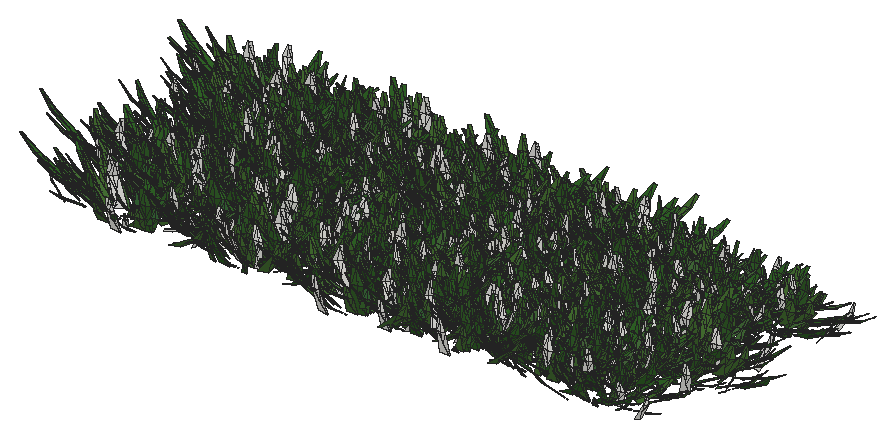
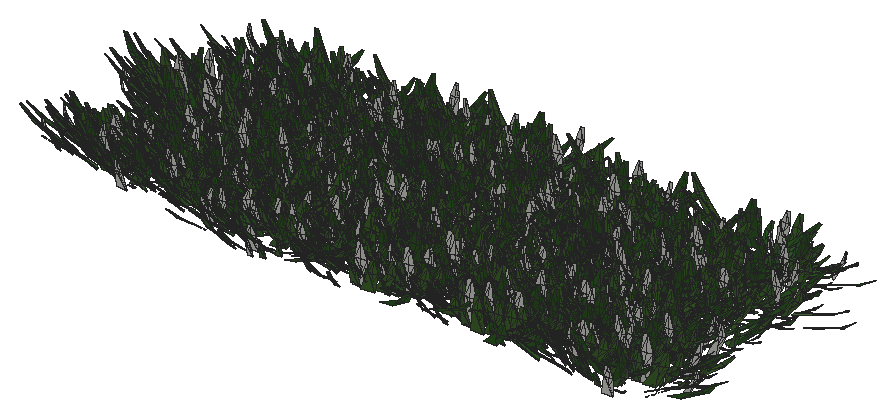
# SketchUp Ruby script. Lengths in inches.
U = 1.inch
M = Sketchup.active_model
def pt(a) = Geom::Point3d.new(a.map { |v| v * U })
def face(e, loops, mat)
  f = e.add_face(loops[0].map { |a| pt(a) })
  loops[1..].each { |l| e.add_face(l.map { |a| pt(a) }).erase! }
  f.material = f.back_material = mat if mat
  f
end
# faces: each face lists its corners as indices into pts; further lists are holes
def faces(e, pts, list, mat = nil) = list.each { |f| face(e, (f[0].is_a?(Array) ? f : [f]).map { |l| l.map { |i| pts[i] } }, mat) }
# xy, xz, yz: faces in a plane at the given z, y or x. An outline is a flat list of corners, or four numbers for a rectangle; further outlines are holes
def ring(l) = l.size == 4 ? [[l[0], l[1]], [l[2], l[1]], [l[2], l[3]], [l[0], l[3]]] : l.each_slice(2).to_a
def flat(e, list, mat, &to3) = list.each { |f| face(e, (f[0].is_a?(Array) ? f : [f]).map { |l| ring(l).map { |u, v| to3.(u, v) } }, mat) }
def xy(e, z, list, mat = nil) = flat(e, list, mat) { |x, y| [x, y, z] }
def xz(e, y, list, mat = nil) = flat(e, list, mat) { |x, z| [x, y, z] }
def yz(e, x, list, mat = nil) = flat(e, list, mat) { |y, z| [x, y, z] }
def lines(e, pts, list) = list.each { |a, b| e.add_line(pt(pts[a]), pt(pts[b])) }
# prism: a flat outline (further loops are holes) pulled along v
def prism(e, loops, v, mat = nil)
  f = face(e, loops, mat); d = Geom::Vector3d.new(v.map { |x| x * U })
  f.pushpull(f.normal.samedirection?(d) ? d.length : -d.length)
end
def box(e, o, s, mat = nil) = prism(e, [[o, [o[0] + s[0], o[1], o[2]], [o[0] + s[0], o[1] + s[1], o[2]], [o[0], o[1] + s[1], o[2]]]], [0, 0, s[2]], mat)
def at(x, y, z, deg = 0) = Geom::Transformation.translation(pt([x, y, z])) * Geom::Transformation.rotation(ORIGIN, Z_AXIS, deg.degrees)
def axes(o, x, y, z) = Geom::Transformation.new([*x, 0, *y, 0, *z, 0, *pt(o).to_a, 1])
def part(name) = M.definitions.add(name)
# library, detail: a bought-in or finely detailed component or shape, given as its bounding box
def library(name, o, s) = part(name).tap { |d| box(d.entities, o, s) }
def detail(e, o, s) = box(e.add_group.entities, o, s)
def put(e, d, t, mat = nil) = e.add_instance(d, t).tap { |i| i.material = mat if mat }
def group(e, t, mat = nil) = e.add_group.tap { |g| g.transformation = t; g.material = mat if mat }.entities
root = M.entities
M.materials.add("Material82").color = [68, 110, 58]
M.materials.add("Material83").color = [48, 90, 38]
M.materials.add("Material84").color = [68, 110, 48]
M.materials.add("Material85").color = [48, 90, 48]
M.materials.add("Material86").color = [58, 110, 58]
M.materials.add("Material87").color = [58, 90, 38]
M.materials.add("Material88").color = [68, 100, 58]
M.materials.add("Material89").color = [48, 100, 38]
c1 = part("grass00")
p = [[-0.6875,0.15,0],[-0.56,0.08,5.52],[-0.04,0.03,2.76],[0.48,-0.02,0],[0.35,-0.02,5.52],[-0.1,-0.14,5.52],
  [-0.12,0.65,8.37],[-0.42,0.65,8.37]]
faces(c1.entities,p,[[0,1,2,3],[3,2,4],[1,5,2],[5,4,2],[1,6,5],[4,5,6],[7,6,1]])
c2 = part("Group16\#1")
put(c2.entities,c1,axes([1.44,-0.61,-0.01],[0.05352,0.12609,0],[-0.10704,0.04543,0.07239],[0.06664,-0.02828,0.11628]),"Material85")
put(c2.entities,c1,axes([0.76,-0.15,-0.01],[0.04676,0.24062,0],[-0.23162,0.04501,0.06642],[0.0652,-0.01267,0.23595]),"Material82")
put(c2.entities,c1,axes([0.79,0.01,-0.01],[-0.00606,0.34651,0],[-0.34381,-0.00602,0.0432],[0.04319,0.00076,0.34386]))
put(c2.entities,c1,axes([1,0.23,-0.01],[-0.07192,0.31144,0],[-0.28722,-0.06632,0.1236],[0.12043,0.02781,0.29478]),"Material84")
put(c2.entities,c1,axes([1.66,0.77,-0.01],[-0.13828,0.29651,0],[-0.21551,-0.1005,0.22471],[0.20365,0.09498,0.23779]),"Material89")
put(c2.entities,c1,axes([0.6875,0.52,-0.01],[-0.18126,0.24051,0],[-0.22746,-0.17142,0.09788],[0.07817,0.05891,0.28481]),"Material84")
put(c2.entities,c1,axes([0.68,0.78,-0.01],[-0.215,0.18688,0],[-0.12385,-0.14248,0.21334],[0.13995,0.16101,0.18878]),"Material82")
put(c2.entities,c1,axes([0.56,1,-0.01],[-0.13756,0.07624,0],[-0.06159,-0.11112,0.0927],[0.04494,0.08108,0.12705]),"Material84")
put(c2.entities,c1,axes([0.2,0.64,-0.01],[-0.23729,0.07254,0],[-0.05711,-0.18681,0.153],[0.04473,0.14632,0.19535]),"Material89")
put(c2.entities,c1,axes([0.0625,0.72,-0.01],[-0.28874,0.02525,0],[-0.02179,-0.24916,0.14647],[0.01276,0.14591,0.25012]),"Material82")
put(c2.entities,c1,axes([-0.08,0.62,-0.01],[-0.34089,-0.04187,0],[0.03255,-0.26504,0.216],[-0.02633,0.21439,0.26703]),"Material89")
put(c2.entities,c1,axes([-0.34,0.98,-0.01],[-0.14314,-0.0493,0],[0.04397,-0.12769,0.06843],[-0.02228,0.0647,0.13505]),"Material89")
put(c2.entities,c1,axes([-0.87,1.45,-0.01],[-0.23488,-0.14114,0],[0.13761,-0.22901,0.06087],[-0.03135,0.05217,0.26717]))
put(c2.entities,c1,axes([-0.72,0.77,-0.01],[-0.14208,-0.13251,0],[0.07209,-0.0773,0.16301],[-0.11118,0.11922,0.1057]),"Material89")
put(c2.entities,c1,axes([-0.62,0.43,-0.01],[-0.14845,-0.21203,0],[0.18654,-0.13061,0.12304],[-0.10079,0.07057,0.22772]),"Material82")
put(c2.entities,c1,axes([-0.68,0.29,-0.01],[-0.13639,-0.32136,0],[0.31723,-0.13464,0.05579],[-0.05136,0.0218,0.34462]),"Material83")
put(c2.entities,c1,axes([-0.64,0.125,-0.01],[-0.0458,-0.23569,0],[0.22124,-0.043,0.08276],[-0.08124,0.01579,0.22538]),"Material86")
put(c2.entities,c1,axes([-1.6,-0.03,-0.01],[0.00576,-0.32897,0],[0.27526,0.00482,0.18018],[-0.18015,-0.00315,0.2753]),"Material84")
put(c2.entities,c1,axes([-1.36,-0.31,-0.01],[0.05718,-0.24765,0],[0.18172,0.04196,0.17267],[-0.16825,-0.03885,0.1865]),"Material89")
put(c2.entities,c1,axes([-1.54,-0.72,-0.01],[0.06537,-0.14017,0],[0.13555,0.06321,0.03939],[-0.0357,-0.01665,0.14956]))
put(c2.entities,c1,axes([-1.19,-0.9,-0.01],[0.09597,-0.12735,0],[0.11214,0.08451,0.07557],[-0.06035,-0.04548,0.14042]),"Material88")
put(c2.entities,c1,axes([-0.47,-0.54,-0.01],[0.11588,-0.10072,0],[0.0618,0.0711,0.12124],[-0.07953,-0.0915,0.0942]))
put(c2.entities,c1,axes([-0.47,-0.84,-0.01],[0.11927,-0.0661,0],[0.06603,0.11913,0.00646],[-0.00313,-0.00565,0.13621]),"Material84")
put(c2.entities,c1,axes([-0.38,-1.24,-0.01],[0.28037,-0.08571,0],[0.0618,0.20215,0.20315],[-0.05939,-0.19428,0.21139]),"Material88")
put(c2.entities,c1,axes([-0.06,-0.66,-0.01],[0.22719,-0.01987,0],[0.01247,0.14255,0.17758],[-0.01547,-0.17691,0.1431]),"Material87")
put(c2.entities,c1,axes([0.11,-0.89,-0.01],[0.14882,0.01828,0],[-0.01058,0.08611,0.12229],[0.01491,-0.12138,0.08676]),"Material85")
put(c2.entities,c1,axes([0.25,-0.72,-0.01],[0.20481,0.07053,0],[-0.06206,0.18022,0.10291],[0.03351,-0.0973,0.1906]),"Material85")
put(c2.entities,c1,axes([0.85,-1.42,-0.01],[0.16481,0.09904,0],[-0.09472,0.15762,0.05616],[0.02893,-0.04814,0.18389]),"Material84")
put(c2.entities,c1,axes([1.01,-1.09,-0.01],[0.21858,0.20385,0],[-0.17495,0.1876,0.15339],[0.10462,-0.11218,0.25652]),"Material89")
put(c2.entities,c1,axes([1.01,-0.71,-0.01],[0.08733,0.12473,0],[-0.06445,0.04512,0.13037],[0.1068,-0.07477,0.07867]),"Material85")
c3 = part("Group15\#1")
put(c3.entities,c2,at(0,0,0))
c4 = part("3darcstudiotree_grass00\#1")
put(c4.entities,c3,at(0,0,0))
put(root,c4,axes([705.6875,346.47,-34.17],[-3.11874,1.35551,0],[-2.91461,-1.04296,-0.0082],[-0.03562,-0.01275,1.73071]))
put(root,c4,axes([707,353.64,-34.17],[-3.23633,-0.50825,0],[1.72306,-1.70642,-0.01803],[0.03469,-0.03435,1.81493]))
put(root,c4,axes([705.92,365.84,-34.17],[-1.77081,1.15286,0],[-3.98211,-0.9513,-0.05645],[-0.27396,-0.06545,1.97994]))
put(root,c4,axes([705.78,364.16,-34.17],[2.97915,0.86965,0],[-2.38175,1.26898,-0.05487],[-0.15774,0.08404,1.44987]))
put(root,c4,axes([707,361.99,-34.17],[3.36447,-1.00796,0],[2.1967,1.14039,-0.03309],[0.10605,0.05506,1.44206]))
put(root,c4,axes([708.45,350.61,-34.17],[-3.57677,-1.09741,0],[2.84767,-1.44352,-0.06227],[0.15089,-0.07649,1.37168]))
put(root,c4,axes([707.32,340.29,-34.17],[-0.9025,1.72738,0],[-3.54084,-0.28772,-0.03296],[-0.16809,-0.01366,1.411]))
put(root,c4,axes([707.48,359.44,-34.17],[-1.59741,1.49736,0],[-3.22806,-0.5356,-0.02216],[-0.12937,-0.02146,1.66252]))
put(root,c4,axes([708.26,348.21,-34.17],[-0.7508,1.54691,0],[-4.43091,-0.33447,-0.01652],[-0.07223,-0.00545,1.50529]))
put(root,c4,axes([708.45,368.2,-34.17],[4.00478,-0.12141,0],[0.32544,1.66956,-0.03486],[0.01415,0.07259,1.68524]))
put(root,c4,axes([708.85,357.11,-34.17],[3.83024,1.03121,0],[-2.22146,1.2833,-0.02215],[-0.08012,0.04629,1.8946]))
put(root,c4,axes([711.74,353.15,-34.17],[-3.68156,-0.36216,0],[0.87025,-1.37591,-0.04204],[0.06138,-0.09705,1.62585]))
put(root,c4,axes([711.4,339.76,-34.17],[-3.79448,1.12109,0],[-2.55555,-1.34526,-0.03017],[-0.0978,-0.05148,1.72726]))
put(root,c4,axes([711.77,363.96,-34.17],[-3.10715,1.0196,0],[-2.89034,-1.36991,-0.01948],[-0.06651,-0.03152,1.80807]))
put(root,c4,axes([711.98,361.45,-34.17],[3.31286,-0.55128,0],[1.80617,1.68812,-0.0407],[0.06877,0.06427,1.51351]))
put(root,c4,axes([711.25,342.87,-34.17],[3.22227,0.82324,0],[-2.17222,1.32236,-0.01048],[-0.0296,0.01802,1.55517]))
put(root,c4,axes([713.39,359.76,-34.17],[-4.269,-0.81813,0],[1.88917,-1.53314,-0.01545],[0.03796,-0.03081,1.8215]))
put(root,c4,axes([712.1,355.12,-34.17],[0.15057,1.31453,0],[-3.70176,0.06595,-0.0329],[-0.23461,0.00418,1.98251]))
put(root,c4,axes([712.07,347.21,-34.17],[-0.68682,1.71759,0],[-4.33467,-0.26958,-0.03641],[-0.15889,-0.00988,1.45326]))
put(root,c4,axes([712.49,348.04,-34.17],[-1.33529,1.77622,0],[-3.16975,-0.37061,-0.00114],[-0.00828,-0.00097,1.86907]))
put(root,c4,axes([712.03,356.7,-34.17],[1.34239,1.63135,0],[-4.02681,0.51535,-0.01715],[-0.07258,0.00929,1.41194]))
put(root,c4,axes([713.12,366.09,-34.17],[-1.89402,1.2029,0],[-3.60721,-0.88336,-0.02009],[-0.09037,-0.02213,1.68525]))
put(root,c4,axes([714.06,350.73,-34.17],[2.81192,0.87479,0],[-2.84329,1.42145,-0.06164],[-0.14998,0.07498,1.3518]))
put(root,c4,axes([714.39,344.07,-34.17],[0.48103,1.53156,0],[-4.51259,0.22043,-0.03401],[-0.13914,0.0068,1.40523]))
put(root,c4,axes([716.875,360.96,-34.17],[-3.65599,0.07986,0],[-0.21877,-1.55768,-0.04105],[-0.01403,-0.0999,1.83253]))
put(root,c4,axes([717.49,350.74,-34.17],[-2.36391,-1.30666,0],[2.88424,-0.81154,-0.04134],[0.24623,-0.06928,1.943]))
put(root,c4,axes([716.77,345.07,-34.17],[-2.91503,0.96344,0],[-2.99535,-1.40954,-0.01682],[-0.05566,-0.02619,1.80026]))
put(root,c4,axes([717.57,349.41,-34.17],[2.5477,-1.31265,0],[2.99582,0.90433,-0.00025],[0.00104,0.00031,1.45509]))
put(root,c4,axes([717.4,363.8125,-34.17],[2.84002,-1.42543,0],[3.17904,0.98511,-0.04001],[0.1906,0.05906,1.83572]))
put(root,c4,axes([716.71,357.56,-34.17],[4.10776,0.45174,0],[-0.96091,1.35899,-0.03867],[-0.06802,0.0962,1.75619]))
put(root,c4,axes([718.67,355.55,-34.17],[-3.02492,-1.16677,0],[2.80082,-1.12934,-0.0483],[0.17838,-0.07192,1.58573]))
put(root,c4,axes([719.11,342.88,-34.17],[1.67083,-1.60234,0],[3.7829,0.6135,-0.00107],[0.00454,0.00074,1.41133]))
put(root,c4,axes([718.7,352.8125,-34.17],[-1.6341,1.38385,0],[-3.29524,-0.60518,-0.01596],[-0.09907,-0.01819,1.86544]))
put(root,c4,axes([718.9375,358.875,-34.17],[-1.88391,1.25543,0],[-3.77395,-0.8808,-0.04665],[-0.1806,-0.04215,1.47851]))
put(root,c4,axes([719.29,346.4375,-34.17],[2.32026,0.93484,0],[-2.86948,1.10768,-0.01876],[-0.07886,0.03044,1.77063]))
put(root,c4,axes([720.03,365.39,-34.17],[0.18236,1.53314,0],[-4.12116,0.07624,-0.04808],[-0.2649,0.0049,1.70557]))
put(root,c4,axes([721.71,352.5,-34.17],[-3.65717,1.04753,0],[-2.10189,-1.14131,-0.02785],[-0.11272,-0.06121,1.84622]))
put(root,c4,axes([721.69,363.99,-34.17],[2.69686,-1.18339,0],[2.47302,0.87653,-0.01288],[0.05957,0.02111,1.54961]))
put(root,c4,axes([722.5625,357.19,-34.17],[-3.84397,-0.38485,0],[1.07963,-1.67717,-0.00944],[0.01366,-0.02122,1.93444]))
put(root,c4,axes([722.41,350.7,-34.17],[-1.0379,-1.53247,0],[3.79206,-0.39944,-0.04991],[0.21721,-0.02288,1.32514]))
put(root,c4,axes([722.54,348.89,-34.17],[1.97874,-1.59829,0],[3.60248,0.69366,-0.03421],[0.19371,0.0373,1.89316]))
put(root,c4,axes([721.76,366.47,-34.17],[1.07752,1.49554,0],[-4.17421,0.46775,-0.01918],[-0.10688,0.01198,1.88463]))
put(root,c4,axes([723.91,346.51,-34.17],[-0.05891,-1.32731,0],[4.1482,-0.02863,-0.04239],[0.194,-0.00134,1.42343]))
put(root,c4,axes([724.71,362.16,-34.17],[-0.12973,-1.5282,0],[4.23676,-0.05594,-0.02714],[0.12341,-0.00163,1.44559]))
put(root,c4,axes([724.33,340.54,-34.17],[2.6038,-1.3441,0],[3.00735,0.90609,-0.00592],[0.02965,0.00893,1.78738]))
put(root,c4,axes([725.1875,341.58,-34.17],[-2.61082,-1.14432,0],[2.90627,-1.03127,-0.02928],[0.10098,-0.03583,1.35967]))
put(root,c4,axes([724.41,367.58,-34.17],[-0.14307,1.431,0],[-4.32963,-0.06732,-0.01193],[-0.07261,-0.00113,1.97773]))
put(root,c4,axes([725.17,355.81,-34.17],[-0.09674,1.30199,0],[-3.40883,-0.03939,-0.04664],[-0.25839,-0.00299,1.41669]))
put(root,c4,axes([725.12,360.35,-34.17],[2.79143,1.2628,0],[-2.51561,0.86486,-0.0286],[-0.15611,0.05367,1.81122]))
put(root,c4,axes([725.36,344.74,-34.17],[-0.55757,1.6642,0],[-4.56304,-0.23777,-0.03274],[-0.13576,-0.00707,1.44297]))
put(root,c4,axes([727.45,359.68,-34.17],[-3.21861,0.39731,0],[-1.33805,-1.68585,-0.0251],[-0.03563,-0.04489,1.59541]))
put(root,c4,axes([727.51,345.94,-34.17],[0.77539,1.49335,0],[-4.15697,0.3357,-0.02758],[-0.13791,0.01114,1.62317]))
put(root,c4,axes([727.78,361.16,-34.17],[0.83918,1.59477,0],[-3.76377,0.30803,-0.00381],[-0.02098,0.00172,1.62105]))
put(root,c4,axes([729.53,354.72,-34.17],[-4.69627,0.21945,0],[-0.46002,-1.53114,-0.03012],[-0.01578,-0.05252,1.30483]))
put(root,c4,axes([728.45,341.91,-34.17],[-1.57534,1.27293,0],[-3.92925,-0.75629,-0.02753],[-0.13899,-0.02675,1.84121]))
put(root,c4,axes([728.83,344.88,-34.17],[2.05797,-1.09603,0],[2.87826,0.84054,-0.04843],[0.25021,0.07307,1.72564]))
put(root,c4,axes([729.86,364.21,-34.17],[1.23956,-1.20185,0],[3.42028,0.54865,-0.0011],[0.00669,0.00107,1.80895]))
put(root,c4,axes([729.91,352.85,-34.17],[0.89327,-1.81074,0],[4.0321,0.30937,-0.02432],[0.12035,0.00923,1.55217]))
put(root,c4,axes([730.79,350.68,-34.17],[0.20119,-1.37174,0],[3.84475,0.0877,-0.03098],[0.16829,0.00384,1.57088]))
put(root,c4,axes([731.14,349.46,-34.17],[-0.37192,-1.4591,0],[3.79295,-0.15037,-0.02999],[0.19954,-0.00791,1.91089]))
put(root,c4,axes([730.87,365.71,-34.17],[2.01038,-1.40201,0],[3.67214,0.81896,-0.04614],[0.18867,0.04208,1.48544]))
put(root,c4,axes([731.11,356.7,-34.17],[4.6177,0.37892,0],[-0.96466,1.82835,-0.01168],[-0.00936,0.01774,1.39591]))
put(root,c4,axes([734.29,362.125,-34.17],[-2.89327,-0.98526,0],[2.3422,-1.06973,-0.01919],[0.0931,-0.04252,1.99409]))
put(root,c4,axes([734.53,347.22,-34.17],[-3.01308,-1.39849,0],[3.33443,-1.11734,-0.06095],[0.24941,-0.08358,1.76096]))
put(root,c4,axes([734.375,351.39,-34.17],[1.17396,-1.50467,0],[4.45897,0.54108,-0.02541],[0.10297,0.01249,1.48254]))
put(root,c4,axes([735.07,357.33,-34.17],[-3.89542,-0.50736,0],[1.22292,-1.46031,-0.04962],[0.09609,-0.11475,1.8049]))
put(root,c4,axes([734.45,349.24,-34.17],[-2.84312,0.65512,0],[-2.18872,-1.47733,-0.05376],[-0.11522,-0.07777,1.38154]))
put(root,c4,axes([733.95,360.03,-34.17],[-0.91872,1.71096,0],[-4.38194,-0.36595,-0.05285],[-0.26515,-0.02214,1.72177]))
put(root,c4,axes([734.6875,342.36,-34.17],[4.14821,-0.06928,0],[0.17152,1.59736,-0.02002],[0.00473,0.044,1.69539]))
put(root,c4,axes([736.54,354.59,-34.17],[-3.82686,-0.23596,0],[0.71117,-1.79387,-0.04342],[0.03245,-0.08186,1.66984]))
put(root,c4,axes([735.47,365.83,-34.17],[-1.95951,1.68141,0],[-3.84767,-0.6974,-0.02861],[-0.15441,-0.02799,1.88512]))
put(root,c4,axes([736.6,352.36,-34.17],[-3.45153,-0.0864,0],[0.28769,-1.78743,-0.04372],[0.01068,-0.06634,1.31241]))
put(root,c4,axes([735.99,363.9,-34.17],[1.28845,1.74913,0],[-3.19455,0.36599,-0.00931],[-0.04886,0.0056,1.3628]))
put(root,c4,axes([736.76,345.01,-34.17],[3.2366,-0.57131,0],[1.58048,1.39258,-0.04939],[0.12568,0.11074,1.80606]))
put(root,c4,axes([738.86,366.41,-34.17],[-3.18632,0.63668,0],[-1.6075,-1.25121,-0.00642],[-0.0144,-0.01121,1.3229]))
put(root,c4,axes([739.48,341.95,-34.17],[-3.56938,-0.43544,0],[1.36231,-1.73682,-0.06046],[0.07694,-0.09809,1.48798]))
put(root,c4,axes([739.02,339.75,-34.17],[-3.08205,1.07293,0],[-3.11637,-1.39229,-0.01862],[-0.0666,-0.02976,1.90809]))
put(root,c4,axes([739,357.74,-34.17],[-2.17882,1.11223,0],[-3.27984,-0.99929,-0.01374],[-0.05934,-0.01808,1.69563]))
put(root,c4,axes([738.66,346.79,-34.17],[-1.12838,1.66356,0],[-4.06225,-0.42855,-0.00132],[-0.00752,-0.00079,1.858]))
put(root,c4,axes([738.27,364.08,-34.17],[3.24771,1.22669,0],[-3.17033,1.30544,-0.01961],[-0.06543,0.02694,1.65716]))
put(root,c4,axes([740.12,344.16,-34.17],[-3.65901,0.17551,0],[-0.56536,-1.83311,-0.00408],[-0.00246,-0.00797,1.74968]))
put(root,c4,axes([738.92,367.59,-34.17],[-1.07809,1.72568,0],[-4.31745,-0.4195,-0.00818],[-0.04348,-0.00422,1.82396]))
put(root,c4,axes([739.84,361.08,-34.17],[2.96136,1.19987,0],[-3.11013,1.19384,-0.004],[-0.01667,0.0064,1.89371]))
put(root,c4,axes([741.65,351.35,-34.17],[-4.14748,0.25836,0],[-0.59761,-1.49206,-0.01239],[-0.00958,-0.02393,1.42361]))
put(root,c4,axes([740.39,348.75,-34.17],[4.21182,0.14848,0],[-0.32581,1.4374,-0.01038],[-0.00654,0.02884,1.94021]))
put(root,c4,axes([740.53,353.38,-34.17],[1.10995,1.51966,0],[-3.58981,0.40779,-0.02733],[-0.15418,0.01751,1.64375]))
put(root,c4,axes([741.7,360.39,-34.17],[4.19014,0.72772,0],[-1.46084,1.30821,-0.04159],[-0.08773,0.07856,1.42181]))
put(root,c4,axes([743.75,348.02,-34.17],[-1.84068,-1.59832,0],[3.91902,-0.70195,-0.02239],[0.11993,-0.02148,1.89813]))
put(root,c4,axes([742.27,354.66,-34.17],[0.99879,1.74855,0],[-3.87665,0.3444,-0.04632],[-0.24296,0.02158,1.6013]))
put(root,c4,axes([745.37,341.84,-34.17],[-0.45548,-1.68091,0],[3.45741,-0.14571,-0.01446],[0.0889,-0.00375,1.61179]))
put(root,c4,axes([744.81,340.49,-34.17],[-3.13157,0.80525,0],[-2.19448,-1.32731,-0.02083],[-0.06068,-0.0367,1.60618]))
put(root,c4,axes([746.07,361.875,-34.17],[-3.37995,-1.26993,0],[3.24999,-1.34532,-0.03405],[0.09733,-0.04029,1.46358]))
put(root,c4,axes([744.1,353.72,-34.17],[1.40547,1.51439,0],[-4.0139,0.57938,-0.03042],[-0.14333,0.02069,1.60735]))
put(root,c4,axes([745.71,346.53,-34.17],[-0.09951,1.54184,0],[-3.8951,-0.0391,-0.03168],[-0.18001,-0.00181,1.66016]))
put(root,c4,axes([746.25,364.19,-34.17],[3.13004,-0.71111,0],[2.12935,1.45771,-0.00508],[0.01244,0.00852,1.56982]))
put(root,c4,axes([745.8125,359.87,-34.17],[1.71903,1.73474,0],[-3.69921,0.57012,-0.05423],[-0.23247,0.03583,1.37014]))
put(root,c4,axes([747.24,355.33,-34.17],[1.52517,-1.72025,0],[3.68343,0.50792,-0.01723],[0.07984,0.01101,1.43549]))
put(root,c4,axes([746.79,344.76,-34.17],[-2.42659,1.57566,0],[-3.75552,-0.89953,-0.06137],[-0.23264,-0.05572,1.46064]))
put(root,c4,axes([746.47,350.39,-34.17],[3.59244,-0.46408,0],[1.16578,1.40355,-0.03684],[0.0661,0.07959,1.61813]))
put(root,c4,axes([747.625,356.9,-34.17],[-3.02925,1.34013,0],[-2.7234,-0.95744,-0.02096],[-0.09613,-0.0338,1.6805]))
put(root,c4,axes([747.48,365.84,-34.17],[2.66376,1.48543,0],[-3.56736,0.99495,-0.03132],[-0.13982,0.039,1.7905]))
put(root,c4,axes([750.49,367.96,-34.17],[-1.65449,-1.67632,0],[3.5536,-0.54549,-0.00938],[0.04968,-0.00763,1.62403]))
put(root,c4,axes([750.6,357.72,-34.17],[-2.10435,-1.3155,0],[3.64518,-0.9069,-0.04882],[0.17684,-0.044,1.38366]))
put(root,c4,axes([749.76,352.34,-34.17],[3.93831,-0.79818,0],[2.14355,1.64496,-0.04443],[0.08068,0.06192,1.39643]))
put(root,c4,axes([751.01,361.03,-34.17],[-2.03778,-1.0951,0],[3.7049,-1.07224,-0.05528],[0.23064,-0.06675,1.78248]))
put(root,c4,axes([751.03,360.06,-34.17],[-3.67688,-0.6634,0],[1.45076,-1.25058,-0.02741],[0.08145,-0.07021,1.86713]))
put(root,c4,axes([749.4,364.18,-34.17],[3.8654,0.35733,0],[-0.81256,1.36706,-0.007],[-0.00937,0.01576,1.56436]))
put(root,c4,axes([751.41,348.66,-34.17],[-3.021,-0.6477,0],[1.60996,-1.16789,-0.02167],[0.0547,-0.03968,1.33527]))
put(root,c4,axes([751.01,340.22,-34.17],[-3.52536,0.66718,0],[-1.57507,-1.29441,-0.02803],[-0.08559,-0.07034,1.92571]))
put(root,c4,axes([750.58,355.35,-34.17],[3.86172,-0.56351,0],[1.21864,1.29888,-0.04569],[0.10723,0.11428,1.78027]))
put(root,c4,axes([751.36,350.49,-34.17],[2.47969,-0.8558,0],[2.79846,1.26111,-0.0129],[0.03707,0.01671,1.39029]))
put(root,c4,axes([751.09,366.86,-34.17],[3.77184,-0.74152,0],[2.04611,1.61872,-0.00236],[0.0043,0.00341,1.40454]))
put(root,c4,axes([751.04,344,-34.17],[4.4523,-0.10128,0],[0.21715,1.4846,-0.03809],[0.01394,0.09529,1.79573]))
put(root,c4,axes([751.47,342.59,-34.17],[3.96943,-0.89247,0],[1.86138,1.2876,-0.05304],[0.17378,0.12021,1.86337]))
put(root,c4,axes([752.89,346.2,-34.17],[-0.06079,-1.40056,0],[3.30003,-0.02228,-0.01279],[0.0855,-0.00058,1.65408]))
put(root,c4,axes([754.83,347.09,-34.17],[-0.30634,-1.35211,0],[4.22133,-0.14875,-0.01785],[0.10663,-0.00376,1.90542]))
put(root,c4,axes([754.91,347.87,-34.17],[0.00917,-1.7323,0],[3.83355,0.00316,-0.00952],[0.04811,0.00004,1.45276]))
put(root,c4,axes([754.86,363.77,-34.17],[3.51422,-0.54071,0],[1.19989,1.21289,-0.03886],[0.08676,0.0877,1.52001]))
put(root,c4,axes([755.65,343.89,-34.17],[0.66388,1.42145,0],[-3.998,0.29041,-0.0472],[-0.22325,0.01622,1.46547]))
put(root,c4,axes([755.76,366.42,-34.17],[2.60904,1.49403,0],[-2.88542,0.78369,-0.04649],[-0.18984,0.05156,1.30192]))
put(root,c4,axes([755.87,354.63,-34.17],[3.83063,0.28141,0],[-0.63066,1.33518,-0.03922],[-0.04064,0.08605,1.46066]))
put(root,c4,axes([758.4,359.01,-34.17],[-2.44222,-1.21448,0],[3.27109,-1.02306,-0.01126],[0.03735,-0.01168,1.32461]))
put(root,c4,axes([758.07,353.71,-34.17],[-3.39135,-0.3159,0],[0.83318,-1.39116,-0.01801],[0.02035,-0.03397,1.33554]))
put(root,c4,axes([757.95,350.4375,-34.17],[-1.25644,-1.35671,0],[3.16457,-0.45581,-0.03784],[0.23357,-0.03364,1.65933]))
put(root,c4,axes([758.51,361.55,-34.17],[-4.6912,-0.24024,0],[0.57575,-1.74859,-0.02421],[0.01544,-0.0469,1.66024]))
put(root,c4,axes([757.62,341.97,-34.17],[3.97766,0.18345,0],[-0.40911,1.37962,-0.0104],[-0.00856,0.02886,1.87036]))
put(root,c4,axes([758.5625,357.85,-34.17],[3.80429,-0.95187,0],[2.21902,1.37934,-0.04672],[0.14892,0.09257,1.84728]))
put(root,c4,axes([760.92,361.2,-34.17],[2.08515,-1.11593,0],[3.14779,0.91479,-0.04551],[0.20545,0.05971,1.64335]))
put(root,c4,axes([760.95,355.11,-34.17],[-2.84594,1.17329,0],[-3.06349,-1.15571,-0.01205],[-0.05136,-0.01938,1.87482]))
put(root,c4,axes([761.98,345.09,-34.17],[-4.1718,-0.04402,0],[0.1133,-1.66995,-0.01377],[0.00192,-0.02825,1.65227]))
put(root,c4,axes([762.5,350.47,-34.17],[-3.23677,-0.61439,0],[2.0349,-1.66734,-0.00367],[0.00726,-0.00595,1.60507]))
put(root,c4,axes([762.11,341.94,-34.17],[0.66157,-1.84804,0],[3.88634,0.21638,-0.01886],[0.11067,0.00616,1.74385]))
put(root,c4,axes([761.125,365.62,-34.17],[3.70848,0.20038,0],[-0.48617,1.3994,-0.00884],[-0.00845,0.02433,1.89082]))
put(root,c4,axes([762.63,348.4375,-34.17],[3.82795,-0.89848,0],[2.12017,1.40489,-0.02674],[0.0662,0.04387,1.50406]))
put(root,c4,axes([763.58,363.38,-34.17],[-3.70161,0.1835,0],[-0.55617,-1.74492,-0.04842],[-0.0352,-0.11043,1.94818]))
put(root,c4,axes([762.78,360.07,-34.17],[4.60425,0.18746,0],[-0.4763,1.81947,-0.06196],[-0.02818,0.10763,1.53928]))
put(root,c4,axes([763,346.01,-34.17],[3.66376,0.25232,0],[-0.75626,1.7079,-0.04039],[-0.02947,0.06656,1.39779]))
put(root,c4,axes([763.25,357.88,-34.17],[3.38223,0.96892,0],[-2.45655,1.33368,-0.05492],[-0.16887,0.09168,1.63919]))
put(root,c4,axes([764.15,353.62,-34.17],[3.17823,1.19717,0],[-2.46254,1.01678,-0.00574],[-0.02103,0.00868,1.41814]))
put(root,c4,axes([767.02,342.06,-34.17],[-4.20115,-0.27572,0],[0.6063,-1.43684,-0.03971],[0.03476,-0.08238,1.4765]))
put(root,c4,axes([766.42,348.79,-34.17],[3.03154,-1.30842,0],[2.70015,0.973,-0.04297],[0.17128,0.06172,1.48019]))
put(root,c4,axes([766.32,351.42,-34.17],[4.0708,-0.43574,0],[1.12817,1.63922,-0.0215],[0.0298,0.0433,1.70776]))
put(root,c4,axes([766.65,362.3125,-34.17],[3.98961,-0.74286,0],[1.49364,1.24762,-0.01833],[0.03992,0.03334,1.33779]))
put(root,c4,axes([766.58,364.36,-34.17],[-1.90909,1.29111,0],[-3.77719,-0.86865,-0.00159],[-0.00678,-0.00156,1.61385]))
put(root,c4,axes([768.64,340.62,-34.17],[-2.56515,-0.8375,0],[2.7288,-1.2999,-0.02106],[0.06081,-0.02897,1.45262]))
put(root,c4,axes([766.62,358.84,-34.17],[1.21271,1.28553,0],[-4.16441,0.61099,-0.01219],[-0.04469,0.00656,1.30286]))
put(root,c4,axes([767.86,352.52,-34.17],[-3.04036,1.06501,0],[-2.34315,-1.04035,-0.02123],[-0.07304,-0.03243,1.37003]))
put(root,c4,axes([768.07,358.19,-34.17],[1.27723,-1.67859,0],[3.60633,0.42678,-0.0465],[0.22987,0.0272,1.45674]))
put(root,c4,axes([767.15,346.06,-34.17],[4.09443,-0.06366,0],[0.15428,1.54325,-0.03451],[0.00867,0.0867,1.8714]))
put(root,c4,axes([767.09,344.07,-34.17],[3.43879,0.48398,0],[-1.47194,1.62658,-0.03925],[-0.05225,0.05774,1.29995]))
put(root,c4,axes([769.5,354.84,-34.17],[-0.06785,-1.57512,0],[4.70678,-0.03153,-0.0635],[0.34719,-0.00233,1.92948]))
put(root,c4,axes([769.95,365.89,-34.17],[3.5964,-0.66598,0],[1.43149,1.20228,-0.03796],[0.09777,0.08212,1.52986]))
put(root,c4,axes([771.89,348.71,-34.17],[-3.83088,0.01586,0],[-0.04003,-1.50367,-0.01485],[-0.00089,-0.03334,1.62647]))
put(root,c4,axes([772.4,362.45,-34.17],[-1.26463,-1.25515,0],[3.81596,-0.59798,-0.04918],[0.19961,-0.03128,1.34418]))
put(root,c4,axes([772.84,364.37,-34.17],[0.54946,-1.30633,0],[4.42126,0.28923,-0.06063],[0.27406,0.01793,1.53907]))
put(root,c4,axes([773.53,352.46,-34.17],[1.45773,-1.41559,0],[3.72691,0.5969,-0.04502],[0.25742,0.04123,1.86083]))
